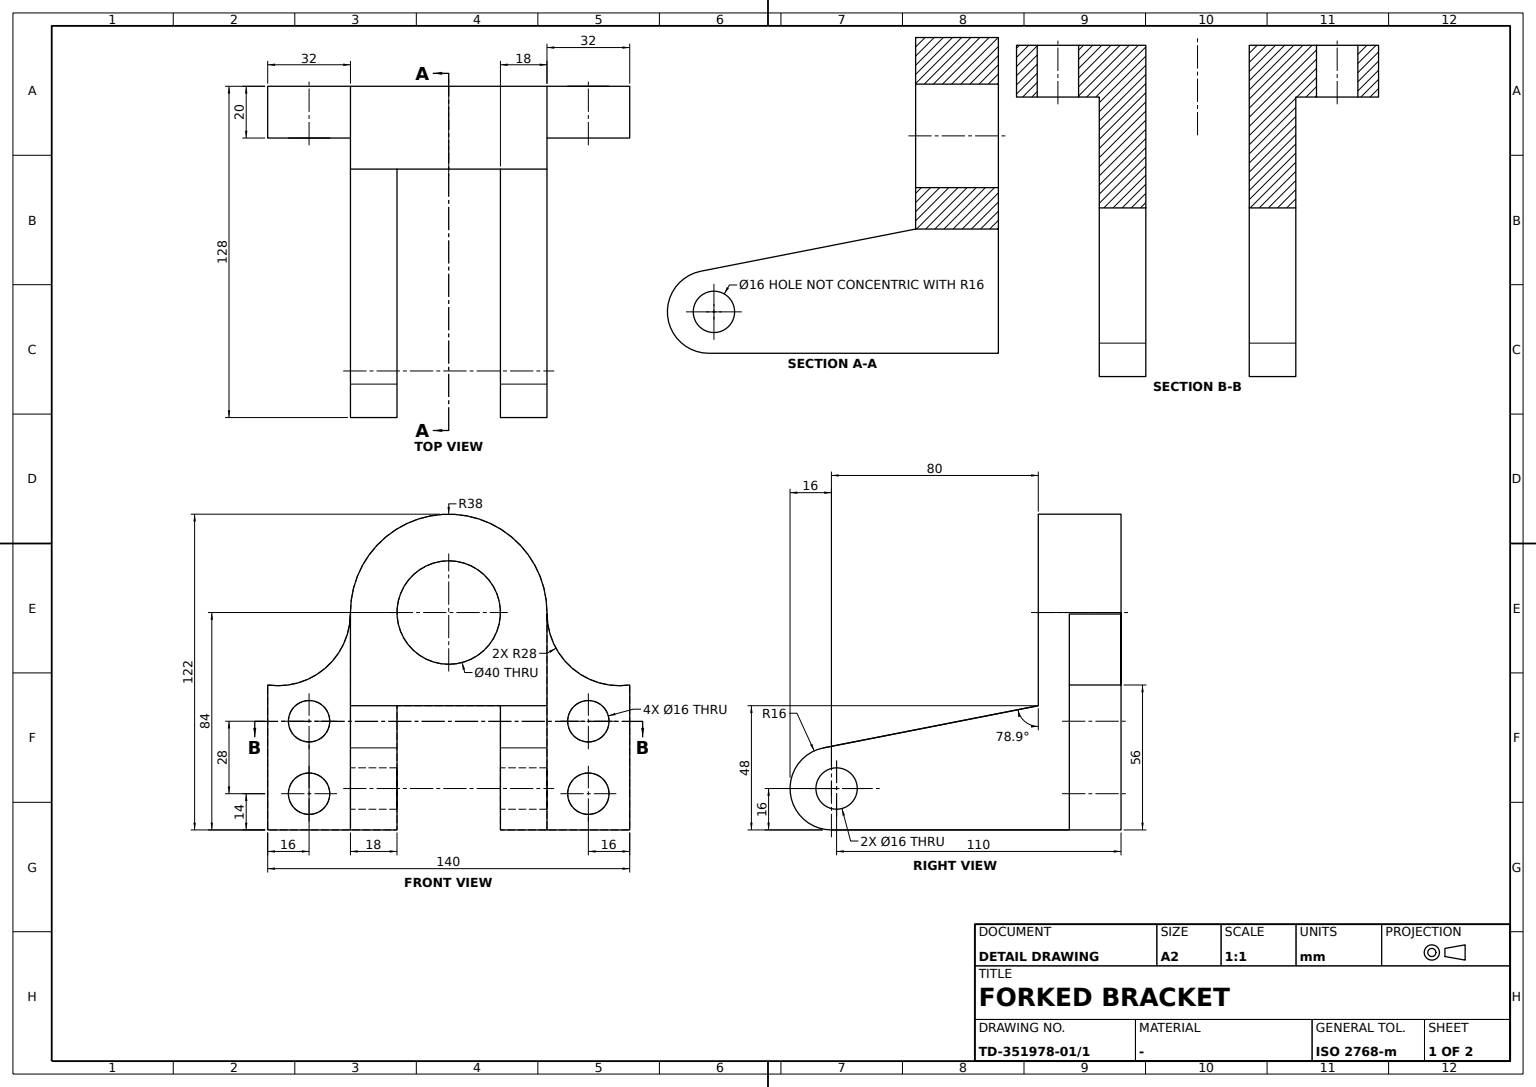
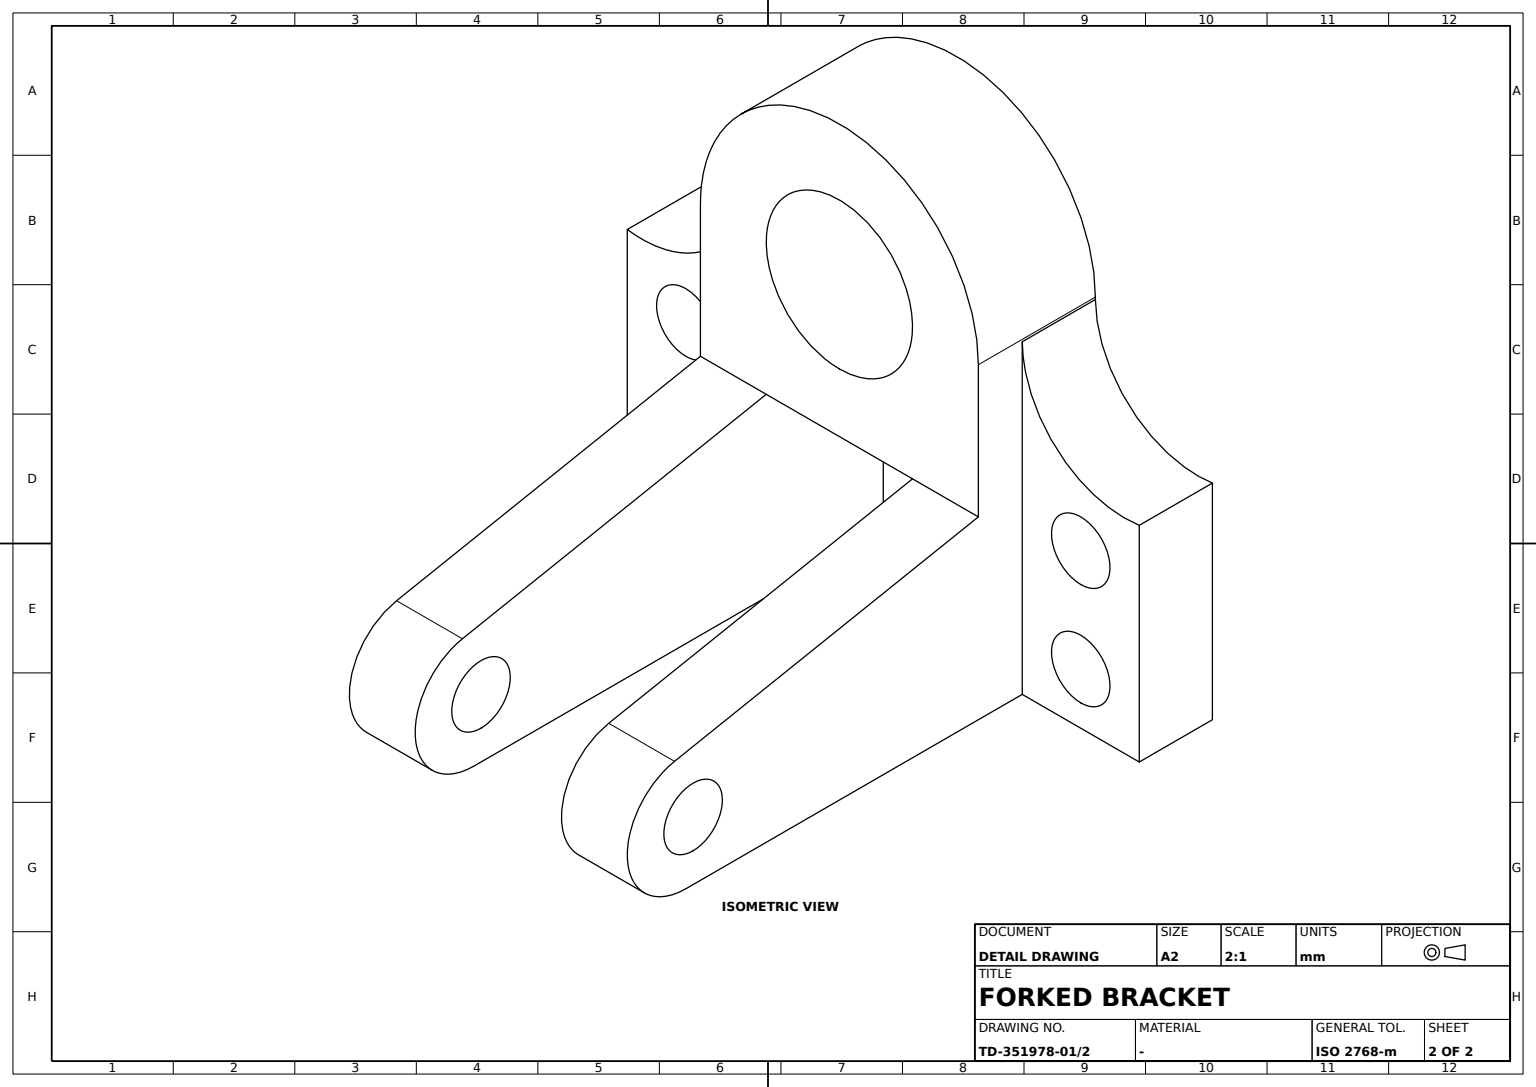
ISO-10303-21;
HEADER;
FILE_DESCRIPTION((''),'2;1');
FILE_NAME('','',(''),(''),'','','');
FILE_SCHEMA(('AUTOMOTIVE_DESIGN'));
ENDSEC;
DATA;
#1=APPLICATION_CONTEXT('');
#2=PRODUCT_CONTEXT('',#1,'mechanical');
#3=PRODUCT('','','',(#2));
#4=PRODUCT_DEFINITION_FORMATION('','',#3);
#5=PRODUCT_DEFINITION_CONTEXT('',#1,'design');
#6=PRODUCT_DEFINITION('','',#4,#5);
#7=PRODUCT_DEFINITION_SHAPE('','',#6);
#8=(LENGTH_UNIT()NAMED_UNIT(*)SI_UNIT(.MILLI.,.METRE.));
#9=(NAMED_UNIT(*)PLANE_ANGLE_UNIT()SI_UNIT($,.RADIAN.));
#10=(NAMED_UNIT(*)SI_UNIT($,.STERADIAN.)SOLID_ANGLE_UNIT());
#11=UNCERTAINTY_MEASURE_WITH_UNIT(LENGTH_MEASURE(0.005),#8,'distance_accuracy_value','');
#12=(GEOMETRIC_REPRESENTATION_CONTEXT(3)GLOBAL_UNCERTAINTY_ASSIGNED_CONTEXT((#11))GLOBAL_UNIT_ASSIGNED_CONTEXT((#8,#9,#10))REPRESENTATION_CONTEXT('',''));
#13=CARTESIAN_POINT('',(94.,-38.,24.));
#14=VERTEX_POINT('',#13);
#15=CARTESIAN_POINT('',(94.,-38.,16.));
#16=DIRECTION('',(0.,1.,0.));
#17=DIRECTION('',(0.,0.,1.));
#18=AXIS2_PLACEMENT_3D('',#15,#16,#17);
#19=CIRCLE('',#18,8.);
#20=EDGE_CURVE('',#14,#14,#19,.F.);
#21=ORIENTED_EDGE('',*,*,#20,.F.);
#22=EDGE_LOOP('',(#21));
#23=FACE_BOUND('',#22,.T.);
#24=CARTESIAN_POINT('',(-16.,-38.,83.425176));
#25=VERTEX_POINT('',#24);
#26=CARTESIAN_POINT('',(-16.,-38.,84.));
#27=VERTEX_POINT('',#26);
#28=CARTESIAN_POINT('',(-16.,-38.,0.));
#29=VECTOR('',#17,1000.);
#30=LINE('',#28,#29);
#31=EDGE_CURVE('',#25,#27,#30,.T.);
#32=ORIENTED_EDGE('',*,*,#31,.F.);
#33=CARTESIAN_POINT('',(4.,-38.,83.425176));
#34=VERTEX_POINT('',#33);
#35=CARTESIAN_POINT('',(-16.,-38.,83.4252));
#36=CARTESIAN_POINT('',(-9.333333,-38.,83.4252));
#37=CARTESIAN_POINT('',(-2.666667,-38.,83.4252));
#38=CARTESIAN_POINT('',(4.,-38.,83.4252));
#39=B_SPLINE_CURVE_WITH_KNOTS('',3,(#35,#36,#37,#38),.UNSPECIFIED.,.F.,.F.,(4,4),(-16.,3.99999975),.UNSPECIFIED.);
#40=EDGE_CURVE('',#25,#34,#39,.T.);
#41=ORIENTED_EDGE('',*,*,#40,.T.);
#42=CARTESIAN_POINT('',(4.,-38.,0.));
#43=VERTEX_POINT('',#42);
#44=DIRECTION('',(0.,0.,-1.));
#45=VECTOR('',#44,1000.);
#46=LINE('',#42,#45);
#47=EDGE_CURVE('',#34,#43,#46,.T.);
#48=ORIENTED_EDGE('',*,*,#47,.T.);
#49=CARTESIAN_POINT('',(96.,-38.,0.));
#50=VERTEX_POINT('',#49);
#51=CARTESIAN_POINT('',(0.,-38.,0.));
#52=DIRECTION('',(1.,0.,0.));
#53=VECTOR('',#52,1000.);
#54=LINE('',#51,#53);
#55=EDGE_CURVE('',#43,#50,#54,.T.);
#56=ORIENTED_EDGE('',*,*,#55,.T.);
#57=CARTESIAN_POINT('',(99.080279,-38.,31.700697));
#58=VERTEX_POINT('',#57);
#59=CARTESIAN_POINT('',(96.,-38.,16.));
#60=AXIS2_PLACEMENT_3D('',#59,#16,#17);
#61=CIRCLE('',#60,16.);
#62=EDGE_CURVE('',#50,#58,#61,.F.);
#63=ORIENTED_EDGE('',*,*,#62,.T.);
#64=CARTESIAN_POINT('',(16.,-38.,48.));
#65=VERTEX_POINT('',#64);
#66=CARTESIAN_POINT('',(9.66098,-38.,49.243636));
#67=DIRECTION('',(-0.981293556,0.,0.192517422));
#68=VECTOR('',#67,1000.);
#69=LINE('',#66,#68);
#70=EDGE_CURVE('',#58,#65,#69,.T.);
#71=ORIENTED_EDGE('',*,*,#70,.T.);
#72=CARTESIAN_POINT('',(16.,-38.,84.));
#73=VERTEX_POINT('',#72);
#74=CARTESIAN_POINT('',(16.,-38.,0.));
#75=LINE('',#74,#29);
#76=EDGE_CURVE('',#65,#73,#75,.T.);
#77=ORIENTED_EDGE('',*,*,#76,.T.);
#78=CARTESIAN_POINT('',(0.,-38.,84.));
#79=LINE('',#78,#53);
#80=EDGE_CURVE('',#73,#27,#79,.F.);
#81=ORIENTED_EDGE('',*,*,#80,.T.);
#82=EDGE_LOOP('',(#32,#41,#48,#56,#63,#71,#77,#81));
#83=FACE_BOUND('',#82,.T.);
#84=AXIS2_PLACEMENT_3D('',#51,#16,#17);
#85=PLANE('',#84);
#86=ADVANCED_FACE('',(#23,#83),#85,.F.);
#87=CARTESIAN_POINT('',(96.,-20.,0.));
#88=VERTEX_POINT('',#87);
#89=CARTESIAN_POINT('',(96.,-29.,0.));
#90=DIRECTION('',(0.,-1.,0.));
#91=VECTOR('',#90,1000.);
#92=LINE('',#89,#91);
#93=EDGE_CURVE('',#50,#88,#92,.F.);
#94=ORIENTED_EDGE('',*,*,#93,.F.);
#95=ORIENTED_EDGE('',*,*,#55,.F.);
#96=CARTESIAN_POINT('',(4.,-70.,0.));
#97=VERTEX_POINT('',#96);
#98=CARTESIAN_POINT('',(4.,-20.,0.));
#99=LINE('',#98,#91);
#100=EDGE_CURVE('',#43,#97,#99,.T.);
#101=ORIENTED_EDGE('',*,*,#100,.T.);
#102=CARTESIAN_POINT('',(-16.,-70.,0.));
#103=VERTEX_POINT('',#102);
#104=LINE('',#102,#53);
#105=EDGE_CURVE('',#103,#97,#104,.T.);
#106=ORIENTED_EDGE('',*,*,#105,.F.);
#107=CARTESIAN_POINT('',(-16.,-20.,0.));
#108=VERTEX_POINT('',#107);
#109=CARTESIAN_POINT('',(-16.,0.,0.));
#110=LINE('',#109,#91);
#111=EDGE_CURVE('',#108,#103,#110,.T.);
#112=ORIENTED_EDGE('',*,*,#111,.F.);
#113=CARTESIAN_POINT('',(0.,-20.,0.));
#114=LINE('',#113,#53);
#115=EDGE_CURVE('',#108,#88,#114,.T.);
#116=ORIENTED_EDGE('',*,*,#115,.T.);
#117=EDGE_LOOP('',(#94,#95,#101,#106,#112,#116));
#118=FACE_BOUND('',#117,.T.);
#119=AXIS2_PLACEMENT_3D('',#113,#17,#90);
#120=PLANE('',#119);
#121=ADVANCED_FACE('',(#118),#120,.F.);
#122=CARTESIAN_POINT('',(99.080279,-20.,31.700697));
#123=VERTEX_POINT('',#122);
#124=CARTESIAN_POINT('',(99.080279,-29.,31.700697));
#125=LINE('',#124,#91);
#126=EDGE_CURVE('',#58,#123,#125,.F.);
#127=ORIENTED_EDGE('',*,*,#126,.T.);
#128=CARTESIAN_POINT('',(16.,-20.,48.));
#129=VERTEX_POINT('',#128);
#130=LINE('',#122,#68);
#131=EDGE_CURVE('',#123,#129,#130,.T.);
#132=ORIENTED_EDGE('',*,*,#131,.T.);
#133=CARTESIAN_POINT('',(16.,0.,48.));
#134=VECTOR('',#16,1000.);
#135=LINE('',#133,#134);
#136=EDGE_CURVE('',#65,#129,#135,.T.);
#137=ORIENTED_EDGE('',*,*,#136,.F.);
#138=ORIENTED_EDGE('',*,*,#70,.F.);
#139=EDGE_LOOP('',(#127,#132,#137,#138));
#140=FACE_BOUND('',#139,.T.);
#141=DIRECTION('',(-0.192517422,0.,-0.981293556));
#142=AXIS2_PLACEMENT_3D('',#57,#141,#67);
#143=PLANE('',#142);
#144=ADVANCED_FACE('',(#140),#143,.F.);
#145=ORIENTED_EDGE('',*,*,#93,.T.);
#146=CARTESIAN_POINT('',(96.,-20.,16.));
#147=AXIS2_PLACEMENT_3D('',#146,#90,#44);
#148=CIRCLE('',#147,16.);
#149=EDGE_CURVE('',#88,#123,#148,.T.);
#150=ORIENTED_EDGE('',*,*,#149,.T.);
#151=ORIENTED_EDGE('',*,*,#126,.F.);
#152=ORIENTED_EDGE('',*,*,#62,.F.);
#153=EDGE_LOOP('',(#145,#150,#151,#152));
#154=FACE_BOUND('',#153,.T.);
#155=CARTESIAN_POINT('',(96.,-29.,16.));
#156=AXIS2_PLACEMENT_3D('',#155,#90,#52);
#157=CYLINDRICAL_SURFACE('',#156,16.);
#158=ADVANCED_FACE('',(#154),#157,.T.);
#159=CARTESIAN_POINT('',(16.,20.,48.));
#160=VERTEX_POINT('',#159);
#161=LINE('',#64,#91);
#162=EDGE_CURVE('',#160,#129,#161,.T.);
#163=ORIENTED_EDGE('',*,*,#162,.T.);
#164=CARTESIAN_POINT('',(-16.,-20.,48.));
#165=VERTEX_POINT('',#164);
#166=CARTESIAN_POINT('',(0.,-20.,48.));
#167=LINE('',#166,#53);
#168=EDGE_CURVE('',#165,#129,#167,.T.);
#169=ORIENTED_EDGE('',*,*,#168,.F.);
#170=CARTESIAN_POINT('',(-16.,20.,48.));
#171=VERTEX_POINT('',#170);
#172=CARTESIAN_POINT('',(-16.,-38.,48.));
#173=LINE('',#172,#91);
#174=EDGE_CURVE('',#171,#165,#173,.T.);
#175=ORIENTED_EDGE('',*,*,#174,.F.);
#176=CARTESIAN_POINT('',(0.,20.,48.));
#177=LINE('',#176,#53);
#178=EDGE_CURVE('',#171,#160,#177,.T.);
#179=ORIENTED_EDGE('',*,*,#178,.T.);
#180=EDGE_LOOP('',(#163,#169,#175,#179));
#181=FACE_BOUND('',#180,.T.);
#182=CARTESIAN_POINT('',(0.,-38.,48.));
#183=AXIS2_PLACEMENT_3D('',#182,#44,#16);
#184=PLANE('',#183);
#185=ADVANCED_FACE('',(#181),#184,.T.);
#186=LINE('',#107,#45);
#187=EDGE_CURVE('',#165,#108,#186,.T.);
#188=ORIENTED_EDGE('',*,*,#187,.F.);
#189=ORIENTED_EDGE('',*,*,#168,.T.);
#190=ORIENTED_EDGE('',*,*,#131,.F.);
#191=ORIENTED_EDGE('',*,*,#149,.F.);
#192=ORIENTED_EDGE('',*,*,#115,.F.);
#193=EDGE_LOOP('',(#188,#189,#190,#191,#192));
#194=FACE_BOUND('',#193,.T.);
#195=CARTESIAN_POINT('',(94.,-20.,8.));
#196=VERTEX_POINT('',#195);
#197=CARTESIAN_POINT('',(94.,-20.,16.));
#198=AXIS2_PLACEMENT_3D('',#197,#90,#44);
#199=CIRCLE('',#198,8.);
#200=EDGE_CURVE('',#196,#196,#199,.T.);
#201=ORIENTED_EDGE('',*,*,#200,.T.);
#202=EDGE_LOOP('',(#201));
#203=FACE_BOUND('',#202,.T.);
#204=AXIS2_PLACEMENT_3D('',#166,#90,#44);
#205=PLANE('',#204);
#206=ADVANCED_FACE('',(#194,#203),#205,.F.);
#207=CARTESIAN_POINT('',(-16.,38.,83.4252));
#208=VERTEX_POINT('',#207);
#209=CARTESIAN_POINT('',(4.,38.,83.425176));
#210=VERTEX_POINT('',#209);
#211=CARTESIAN_POINT('',(4.,38.,83.4252));
#212=CARTESIAN_POINT('',(-2.666667,38.,83.4252));
#213=CARTESIAN_POINT('',(-9.333333,38.,83.4252));
#214=B_SPLINE_CURVE_WITH_KNOTS('',3,(#211,#212,#213,#207),.UNSPECIFIED.,.F.,.F.,(4,4),(-15.99999975,3.999999833),.UNSPECIFIED.);
#215=EDGE_CURVE('',#208,#210,#214,.F.);
#216=ORIENTED_EDGE('',*,*,#215,.T.);
#217=CARTESIAN_POINT('',(4.,70.,55.999787));
#218=VERTEX_POINT('',#217);
#219=CARTESIAN_POINT('',(4.,66.,83.7126));
#220=DIRECTION('',(-1.,0.,0.));
#221=AXIS2_PLACEMENT_3D('',#219,#220,#17);
#222=CIRCLE('',#221,28.);
#223=EDGE_CURVE('',#210,#218,#222,.F.);
#224=ORIENTED_EDGE('',*,*,#223,.T.);
#225=CARTESIAN_POINT('',(-16.,70.,55.999787));
#226=VERTEX_POINT('',#225);
#227=LINE('',#225,#53);
#228=EDGE_CURVE('',#226,#218,#227,.T.);
#229=ORIENTED_EDGE('',*,*,#228,.F.);
#230=CARTESIAN_POINT('',(-16.,66.,83.7126));
#231=AXIS2_PLACEMENT_3D('',#230,#52,#44);
#232=CIRCLE('',#231,28.);
#233=EDGE_CURVE('',#208,#226,#232,.T.);
#234=ORIENTED_EDGE('',*,*,#233,.F.);
#235=EDGE_LOOP('',(#216,#224,#229,#234));
#236=FACE_BOUND('',#235,.T.);
#237=CARTESIAN_POINT('',(-6.,66.,83.7126));
#238=AXIS2_PLACEMENT_3D('',#237,#52,#16);
#239=CYLINDRICAL_SURFACE('',#238,28.);
#240=ADVANCED_FACE('',(#236),#239,.F.);
#241=CARTESIAN_POINT('',(4.,54.,22.));
#242=VERTEX_POINT('',#241);
#243=CARTESIAN_POINT('',(4.,54.,14.));
#244=AXIS2_PLACEMENT_3D('',#243,#220,#17);
#245=CIRCLE('',#244,8.);
#246=EDGE_CURVE('',#242,#242,#245,.T.);
#247=ORIENTED_EDGE('',*,*,#246,.F.);
#248=EDGE_LOOP('',(#247));
#249=FACE_BOUND('',#248,.T.);
#250=CARTESIAN_POINT('',(-16.,54.,6.));
#251=VERTEX_POINT('',#250);
#252=CARTESIAN_POINT('',(-16.,54.,14.));
#253=AXIS2_PLACEMENT_3D('',#252,#52,#44);
#254=CIRCLE('',#253,8.);
#255=EDGE_CURVE('',#251,#251,#254,.F.);
#256=ORIENTED_EDGE('',*,*,#255,.T.);
#257=EDGE_LOOP('',(#256));
#258=FACE_BOUND('',#257,.T.);
#259=CARTESIAN_POINT('',(-6.,54.,14.));
#260=AXIS2_PLACEMENT_3D('',#259,#220,#90);
#261=CYLINDRICAL_SURFACE('',#260,8.);
#262=ADVANCED_FACE('',(#249,#258),#261,.F.);
#263=CARTESIAN_POINT('',(96.,20.,0.));
#264=VERTEX_POINT('',#263);
#265=CARTESIAN_POINT('',(99.080279,20.,31.700697));
#266=VERTEX_POINT('',#265);
#267=CARTESIAN_POINT('',(96.,20.,16.));
#268=AXIS2_PLACEMENT_3D('',#267,#16,#17);
#269=CIRCLE('',#268,16.);
#270=EDGE_CURVE('',#264,#266,#269,.F.);
#271=ORIENTED_EDGE('',*,*,#270,.F.);
#272=CARTESIAN_POINT('',(96.,38.,0.));
#273=VERTEX_POINT('',#272);
#274=EDGE_CURVE('',#273,#264,#92,.T.);
#275=ORIENTED_EDGE('',*,*,#274,.F.);
#276=CARTESIAN_POINT('',(99.080279,38.,31.700697));
#277=VERTEX_POINT('',#276);
#278=CARTESIAN_POINT('',(96.,38.,16.));
#279=AXIS2_PLACEMENT_3D('',#278,#90,#44);
#280=CIRCLE('',#279,16.);
#281=EDGE_CURVE('',#273,#277,#280,.T.);
#282=ORIENTED_EDGE('',*,*,#281,.T.);
#283=EDGE_CURVE('',#277,#266,#125,.T.);
#284=ORIENTED_EDGE('',*,*,#283,.T.);
#285=EDGE_LOOP('',(#271,#275,#282,#284));
#286=FACE_BOUND('',#285,.T.);
#287=ADVANCED_FACE('',(#286),#157,.T.);
#288=ORIENTED_EDGE('',*,*,#105,.T.);
#289=CARTESIAN_POINT('',(4.,-70.,55.999787));
#290=VERTEX_POINT('',#289);
#291=LINE('',#96,#29);
#292=EDGE_CURVE('',#97,#290,#291,.T.);
#293=ORIENTED_EDGE('',*,*,#292,.T.);
#294=CARTESIAN_POINT('',(-16.,-70.,55.999787));
#295=VERTEX_POINT('',#294);
#296=VECTOR('',#220,1000.);
#297=LINE('',#294,#296);
#298=EDGE_CURVE('',#295,#290,#297,.F.);
#299=ORIENTED_EDGE('',*,*,#298,.F.);
#300=LINE('',#102,#29);
#301=EDGE_CURVE('',#103,#295,#300,.T.);
#302=ORIENTED_EDGE('',*,*,#301,.F.);
#303=EDGE_LOOP('',(#288,#293,#299,#302));
#304=FACE_BOUND('',#303,.T.);
#305=AXIS2_PLACEMENT_3D('',#102,#16,#17);
#306=PLANE('',#305);
#307=ADVANCED_FACE('',(#304),#306,.F.);
#308=CARTESIAN_POINT('',(94.,20.,24.));
#309=VERTEX_POINT('',#308);
#310=CARTESIAN_POINT('',(94.,20.,16.));
#311=AXIS2_PLACEMENT_3D('',#310,#16,#17);
#312=CIRCLE('',#311,8.);
#313=EDGE_CURVE('',#309,#309,#312,.T.);
#314=ORIENTED_EDGE('',*,*,#313,.F.);
#315=EDGE_LOOP('',(#314));
#316=FACE_BOUND('',#315,.T.);
#317=CARTESIAN_POINT('',(94.,38.,8.));
#318=VERTEX_POINT('',#317);
#319=CARTESIAN_POINT('',(94.,38.,16.));
#320=AXIS2_PLACEMENT_3D('',#319,#90,#44);
#321=CIRCLE('',#320,8.);
#322=EDGE_CURVE('',#318,#318,#321,.T.);
#323=ORIENTED_EDGE('',*,*,#322,.F.);
#324=EDGE_LOOP('',(#323));
#325=FACE_BOUND('',#324,.T.);
#326=CARTESIAN_POINT('',(94.,6.5,16.));
#327=AXIS2_PLACEMENT_3D('',#326,#90,#52);
#328=CYLINDRICAL_SURFACE('',#327,8.);
#329=ADVANCED_FACE('',(#316,#325),#328,.F.);
#330=CARTESIAN_POINT('',(-16.,54.,34.));
#331=VERTEX_POINT('',#330);
#332=CARTESIAN_POINT('',(-16.,54.,42.));
#333=AXIS2_PLACEMENT_3D('',#332,#52,#44);
#334=CIRCLE('',#333,8.);
#335=EDGE_CURVE('',#331,#331,#334,.F.);
#336=ORIENTED_EDGE('',*,*,#335,.T.);
#337=EDGE_LOOP('',(#336));
#338=FACE_BOUND('',#337,.T.);
#339=CARTESIAN_POINT('',(4.,54.,50.));
#340=VERTEX_POINT('',#339);
#341=CARTESIAN_POINT('',(4.,54.,42.));
#342=AXIS2_PLACEMENT_3D('',#341,#220,#17);
#343=CIRCLE('',#342,8.);
#344=EDGE_CURVE('',#340,#340,#343,.T.);
#345=ORIENTED_EDGE('',*,*,#344,.F.);
#346=EDGE_LOOP('',(#345));
#347=FACE_BOUND('',#346,.T.);
#348=CARTESIAN_POINT('',(-6.,54.,42.));
#349=AXIS2_PLACEMENT_3D('',#348,#220,#90);
#350=CYLINDRICAL_SURFACE('',#349,8.);
#351=ADVANCED_FACE('',(#338,#347),#350,.F.);
#352=CARTESIAN_POINT('',(16.,0.,64.));
#353=VERTEX_POINT('',#352);
#354=CARTESIAN_POINT('',(16.,0.,84.));
#355=AXIS2_PLACEMENT_3D('',#354,#52,#44);
#356=CIRCLE('',#355,20.);
#357=EDGE_CURVE('',#353,#353,#356,.T.);
#358=ORIENTED_EDGE('',*,*,#357,.T.);
#359=EDGE_LOOP('',(#358));
#360=FACE_BOUND('',#359,.T.);
#361=CARTESIAN_POINT('',(-16.,0.,64.));
#362=VERTEX_POINT('',#361);
#363=CARTESIAN_POINT('',(-16.,0.,84.));
#364=AXIS2_PLACEMENT_3D('',#363,#52,#44);
#365=CIRCLE('',#364,20.);
#366=EDGE_CURVE('',#362,#362,#365,.T.);
#367=ORIENTED_EDGE('',*,*,#366,.F.);
#368=EDGE_LOOP('',(#367));
#369=FACE_BOUND('',#368,.T.);
#370=CARTESIAN_POINT('',(0.,0.,84.));
#371=AXIS2_PLACEMENT_3D('',#370,#52,#16);
#372=CYLINDRICAL_SURFACE('',#371,20.);
#373=ADVANCED_FACE('',(#360,#369),#372,.F.);
#374=CARTESIAN_POINT('',(16.,38.,48.));
#375=VERTEX_POINT('',#374);
#376=EDGE_CURVE('',#375,#160,#161,.T.);
#377=ORIENTED_EDGE('',*,*,#376,.T.);
#378=CARTESIAN_POINT('',(9.66098,20.,49.243636));
#379=LINE('',#378,#68);
#380=EDGE_CURVE('',#266,#160,#379,.T.);
#381=ORIENTED_EDGE('',*,*,#380,.F.);
#382=ORIENTED_EDGE('',*,*,#283,.F.);
#383=LINE('',#276,#68);
#384=EDGE_CURVE('',#277,#375,#383,.T.);
#385=ORIENTED_EDGE('',*,*,#384,.T.);
#386=EDGE_LOOP('',(#377,#381,#382,#385));
#387=FACE_BOUND('',#386,.T.);
#388=ADVANCED_FACE('',(#387),#143,.F.);
#389=CARTESIAN_POINT('',(-16.,70.,0.));
#390=VERTEX_POINT('',#389);
#391=CARTESIAN_POINT('',(4.,70.,0.));
#392=VERTEX_POINT('',#391);
#393=LINE('',#389,#53);
#394=EDGE_CURVE('',#390,#392,#393,.T.);
#395=ORIENTED_EDGE('',*,*,#394,.F.);
#396=LINE('',#389,#29);
#397=EDGE_CURVE('',#390,#226,#396,.T.);
#398=ORIENTED_EDGE('',*,*,#397,.T.);
#399=ORIENTED_EDGE('',*,*,#228,.T.);
#400=LINE('',#391,#29);
#401=EDGE_CURVE('',#392,#218,#400,.T.);
#402=ORIENTED_EDGE('',*,*,#401,.F.);
#403=EDGE_LOOP('',(#395,#398,#399,#402));
#404=FACE_BOUND('',#403,.T.);
#405=AXIS2_PLACEMENT_3D('',#389,#16,#17);
#406=PLANE('',#405);
#407=ADVANCED_FACE('',(#404),#406,.T.);
#408=CARTESIAN_POINT('',(4.,38.,0.));
#409=VERTEX_POINT('',#408);
#410=CARTESIAN_POINT('',(4.,38.,48.));
#411=LINE('',#410,#45);
#412=EDGE_CURVE('',#210,#409,#411,.T.);
#413=ORIENTED_EDGE('',*,*,#412,.T.);
#414=CARTESIAN_POINT('',(4.,0.,0.));
#415=LINE('',#414,#134);
#416=EDGE_CURVE('',#409,#392,#415,.T.);
#417=ORIENTED_EDGE('',*,*,#416,.T.);
#418=ORIENTED_EDGE('',*,*,#401,.T.);
#419=ORIENTED_EDGE('',*,*,#223,.F.);
#420=EDGE_LOOP('',(#413,#417,#418,#419));
#421=FACE_BOUND('',#420,.T.);
#422=ORIENTED_EDGE('',*,*,#344,.T.);
#423=EDGE_LOOP('',(#422));
#424=FACE_BOUND('',#423,.T.);
#425=ORIENTED_EDGE('',*,*,#246,.T.);
#426=EDGE_LOOP('',(#425));
#427=FACE_BOUND('',#426,.T.);
#428=AXIS2_PLACEMENT_3D('',#414,#220,#90);
#429=PLANE('',#428);
#430=ADVANCED_FACE('',(#421,#424,#427),#429,.F.);
#431=ORIENTED_EDGE('',*,*,#274,.T.);
#432=CARTESIAN_POINT('',(-16.,20.,0.));
#433=VERTEX_POINT('',#432);
#434=CARTESIAN_POINT('',(0.,20.,0.));
#435=LINE('',#434,#53);
#436=EDGE_CURVE('',#433,#264,#435,.T.);
#437=ORIENTED_EDGE('',*,*,#436,.F.);
#438=EDGE_CURVE('',#390,#433,#110,.T.);
#439=ORIENTED_EDGE('',*,*,#438,.F.);
#440=ORIENTED_EDGE('',*,*,#394,.T.);
#441=ORIENTED_EDGE('',*,*,#416,.F.);
#442=CARTESIAN_POINT('',(0.,38.,0.));
#443=LINE('',#442,#53);
#444=EDGE_CURVE('',#409,#273,#443,.T.);
#445=ORIENTED_EDGE('',*,*,#444,.T.);
#446=EDGE_LOOP('',(#431,#437,#439,#440,#441,#445));
#447=FACE_BOUND('',#446,.T.);
#448=ADVANCED_FACE('',(#447),#120,.F.);
#449=ORIENTED_EDGE('',*,*,#40,.F.);
#450=CARTESIAN_POINT('',(-16.,-66.,83.7126));
#451=AXIS2_PLACEMENT_3D('',#450,#52,#44);
#452=CIRCLE('',#451,28.);
#453=EDGE_CURVE('',#25,#295,#452,.F.);
#454=ORIENTED_EDGE('',*,*,#453,.T.);
#455=ORIENTED_EDGE('',*,*,#298,.T.);
#456=CARTESIAN_POINT('',(4.,-66.,83.7126));
#457=AXIS2_PLACEMENT_3D('',#456,#220,#17);
#458=CIRCLE('',#457,28.);
#459=EDGE_CURVE('',#34,#290,#458,.T.);
#460=ORIENTED_EDGE('',*,*,#459,.F.);
#461=EDGE_LOOP('',(#449,#454,#455,#460));
#462=FACE_BOUND('',#461,.T.);
#463=CARTESIAN_POINT('',(-6.,-66.,83.7126));
#464=AXIS2_PLACEMENT_3D('',#463,#220,#90);
#465=CYLINDRICAL_SURFACE('',#464,28.);
#466=ADVANCED_FACE('',(#462),#465,.F.);
#467=ORIENTED_EDGE('',*,*,#162,.F.);
#468=ORIENTED_EDGE('',*,*,#376,.F.);
#469=CARTESIAN_POINT('',(16.,38.,84.));
#470=VERTEX_POINT('',#469);
#471=CARTESIAN_POINT('',(16.,38.,0.));
#472=LINE('',#471,#45);
#473=EDGE_CURVE('',#470,#375,#472,.T.);
#474=ORIENTED_EDGE('',*,*,#473,.F.);
#475=CIRCLE('',#355,38.);
#476=EDGE_CURVE('',#470,#73,#475,.T.);
#477=ORIENTED_EDGE('',*,*,#476,.T.);
#478=ORIENTED_EDGE('',*,*,#76,.F.);
#479=ORIENTED_EDGE('',*,*,#136,.T.);
#480=EDGE_LOOP('',(#467,#468,#474,#477,#478,#479));
#481=FACE_BOUND('',#480,.T.);
#482=ORIENTED_EDGE('',*,*,#357,.F.);
#483=EDGE_LOOP('',(#482));
#484=FACE_BOUND('',#483,.T.);
#485=CARTESIAN_POINT('',(16.,0.,0.));
#486=AXIS2_PLACEMENT_3D('',#485,#52,#16);
#487=PLANE('',#486);
#488=ADVANCED_FACE('',(#481,#484),#487,.T.);
#489=ORIENTED_EDGE('',*,*,#80,.F.);
#490=ORIENTED_EDGE('',*,*,#476,.F.);
#491=CARTESIAN_POINT('',(-16.,38.,84.));
#492=VERTEX_POINT('',#491);
#493=CARTESIAN_POINT('',(0.,38.,84.));
#494=LINE('',#493,#53);
#495=EDGE_CURVE('',#470,#492,#494,.F.);
#496=ORIENTED_EDGE('',*,*,#495,.T.);
#497=CIRCLE('',#364,38.);
#498=EDGE_CURVE('',#492,#27,#497,.T.);
#499=ORIENTED_EDGE('',*,*,#498,.T.);
#500=EDGE_LOOP('',(#489,#490,#496,#499));
#501=FACE_BOUND('',#500,.T.);
#502=CYLINDRICAL_SURFACE('',#371,38.);
#503=ADVANCED_FACE('',(#501),#502,.T.);
#504=ORIENTED_EDGE('',*,*,#495,.F.);
#505=ORIENTED_EDGE('',*,*,#473,.T.);
#506=ORIENTED_EDGE('',*,*,#384,.F.);
#507=ORIENTED_EDGE('',*,*,#281,.F.);
#508=ORIENTED_EDGE('',*,*,#444,.F.);
#509=ORIENTED_EDGE('',*,*,#412,.F.);
#510=ORIENTED_EDGE('',*,*,#215,.F.);
#511=CARTESIAN_POINT('',(-16.,38.,0.));
#512=LINE('',#511,#45);
#513=EDGE_CURVE('',#492,#208,#512,.T.);
#514=ORIENTED_EDGE('',*,*,#513,.F.);
#515=EDGE_LOOP('',(#504,#505,#506,#507,#508,#509,#510,#514));
#516=FACE_BOUND('',#515,.T.);
#517=ORIENTED_EDGE('',*,*,#322,.T.);
#518=EDGE_LOOP('',(#517));
#519=FACE_BOUND('',#518,.T.);
#520=CARTESIAN_POINT('',(0.,38.,48.));
#521=AXIS2_PLACEMENT_3D('',#520,#90,#44);
#522=PLANE('',#521);
#523=ADVANCED_FACE('',(#516,#519),#522,.F.);
#524=ORIENTED_EDGE('',*,*,#255,.F.);
#525=EDGE_LOOP('',(#524));
#526=FACE_BOUND('',#525,.T.);
#527=ORIENTED_EDGE('',*,*,#513,.T.);
#528=ORIENTED_EDGE('',*,*,#233,.T.);
#529=ORIENTED_EDGE('',*,*,#397,.F.);
#530=ORIENTED_EDGE('',*,*,#438,.T.);
#531=LINE('',#432,#29);
#532=EDGE_CURVE('',#433,#171,#531,.T.);
#533=ORIENTED_EDGE('',*,*,#532,.T.);
#534=ORIENTED_EDGE('',*,*,#174,.T.);
#535=ORIENTED_EDGE('',*,*,#187,.T.);
#536=ORIENTED_EDGE('',*,*,#111,.T.);
#537=ORIENTED_EDGE('',*,*,#301,.T.);
#538=ORIENTED_EDGE('',*,*,#453,.F.);
#539=ORIENTED_EDGE('',*,*,#31,.T.);
#540=ORIENTED_EDGE('',*,*,#498,.F.);
#541=EDGE_LOOP('',(#527,#528,#529,#530,#533,#534,#535,#536,#537,#538,#539,#540));
#542=FACE_BOUND('',#541,.T.);
#543=CARTESIAN_POINT('',(-16.,-54.,6.));
#544=VERTEX_POINT('',#543);
#545=CARTESIAN_POINT('',(-16.,-54.,14.));
#546=AXIS2_PLACEMENT_3D('',#545,#52,#44);
#547=CIRCLE('',#546,8.);
#548=EDGE_CURVE('',#544,#544,#547,.T.);
#549=ORIENTED_EDGE('',*,*,#548,.T.);
#550=EDGE_LOOP('',(#549));
#551=FACE_BOUND('',#550,.T.);
#552=ORIENTED_EDGE('',*,*,#335,.F.);
#553=EDGE_LOOP('',(#552));
#554=FACE_BOUND('',#553,.T.);
#555=CARTESIAN_POINT('',(-16.,-54.,34.));
#556=VERTEX_POINT('',#555);
#557=CARTESIAN_POINT('',(-16.,-54.,42.));
#558=AXIS2_PLACEMENT_3D('',#557,#52,#44);
#559=CIRCLE('',#558,8.);
#560=EDGE_CURVE('',#556,#556,#559,.T.);
#561=ORIENTED_EDGE('',*,*,#560,.T.);
#562=EDGE_LOOP('',(#561));
#563=FACE_BOUND('',#562,.T.);
#564=ORIENTED_EDGE('',*,*,#366,.T.);
#565=EDGE_LOOP('',(#564));
#566=FACE_BOUND('',#565,.T.);
#567=AXIS2_PLACEMENT_3D('',#109,#52,#16);
#568=PLANE('',#567);
#569=ADVANCED_FACE('',(#526,#542,#551,#554,#563,#566),#568,.F.);
#570=ORIENTED_EDGE('',*,*,#200,.F.);
#571=EDGE_LOOP('',(#570));
#572=FACE_BOUND('',#571,.T.);
#573=ORIENTED_EDGE('',*,*,#20,.T.);
#574=EDGE_LOOP('',(#573));
#575=FACE_BOUND('',#574,.T.);
#576=ADVANCED_FACE('',(#572,#575),#328,.F.);
#577=ORIENTED_EDGE('',*,*,#560,.F.);
#578=EDGE_LOOP('',(#577));
#579=FACE_BOUND('',#578,.T.);
#580=CARTESIAN_POINT('',(4.,-54.,50.));
#581=VERTEX_POINT('',#580);
#582=CARTESIAN_POINT('',(4.,-54.,42.));
#583=AXIS2_PLACEMENT_3D('',#582,#220,#17);
#584=CIRCLE('',#583,8.);
#585=EDGE_CURVE('',#581,#581,#584,.F.);
#586=ORIENTED_EDGE('',*,*,#585,.T.);
#587=EDGE_LOOP('',(#586));
#588=FACE_BOUND('',#587,.T.);
#589=CARTESIAN_POINT('',(-6.,-54.,42.));
#590=AXIS2_PLACEMENT_3D('',#589,#52,#16);
#591=CYLINDRICAL_SURFACE('',#590,8.);
#592=ADVANCED_FACE('',(#579,#588),#591,.F.);
#593=ORIENTED_EDGE('',*,*,#548,.F.);
#594=EDGE_LOOP('',(#593));
#595=FACE_BOUND('',#594,.T.);
#596=CARTESIAN_POINT('',(4.,-54.,22.));
#597=VERTEX_POINT('',#596);
#598=CARTESIAN_POINT('',(4.,-54.,14.));
#599=AXIS2_PLACEMENT_3D('',#598,#220,#17);
#600=CIRCLE('',#599,8.);
#601=EDGE_CURVE('',#597,#597,#600,.F.);
#602=ORIENTED_EDGE('',*,*,#601,.T.);
#603=EDGE_LOOP('',(#602));
#604=FACE_BOUND('',#603,.T.);
#605=CARTESIAN_POINT('',(-6.,-54.,14.));
#606=AXIS2_PLACEMENT_3D('',#605,#52,#16);
#607=CYLINDRICAL_SURFACE('',#606,8.);
#608=ADVANCED_FACE('',(#595,#604),#607,.F.);
#609=ORIENTED_EDGE('',*,*,#585,.F.);
#610=EDGE_LOOP('',(#609));
#611=FACE_BOUND('',#610,.T.);
#612=ORIENTED_EDGE('',*,*,#601,.F.);
#613=EDGE_LOOP('',(#612));
#614=FACE_BOUND('',#613,.T.);
#615=ORIENTED_EDGE('',*,*,#100,.F.);
#616=ORIENTED_EDGE('',*,*,#47,.F.);
#617=ORIENTED_EDGE('',*,*,#459,.T.);
#618=ORIENTED_EDGE('',*,*,#292,.F.);
#619=EDGE_LOOP('',(#615,#616,#617,#618));
#620=FACE_BOUND('',#619,.T.);
#621=ADVANCED_FACE('',(#611,#614,#620),#429,.F.);
#622=ORIENTED_EDGE('',*,*,#313,.T.);
#623=EDGE_LOOP('',(#622));
#624=FACE_BOUND('',#623,.T.);
#625=ORIENTED_EDGE('',*,*,#380,.T.);
#626=ORIENTED_EDGE('',*,*,#178,.F.);
#627=ORIENTED_EDGE('',*,*,#532,.F.);
#628=ORIENTED_EDGE('',*,*,#436,.T.);
#629=ORIENTED_EDGE('',*,*,#270,.T.);
#630=EDGE_LOOP('',(#625,#626,#627,#628,#629));
#631=FACE_BOUND('',#630,.T.);
#632=AXIS2_PLACEMENT_3D('',#434,#16,#17);
#633=PLANE('',#632);
#634=ADVANCED_FACE('',(#624,#631),#633,.F.);
#635=CLOSED_SHELL('',(#86,#121,#144,#158,#185,#206,#240,#262,#287,#307,#329,#351,#373,#388,#407,#430,#448,#466,#488,#503,#523,#569,#576,#592,#608,#621,#634));
#636=MANIFOLD_SOLID_BREP('',#635);
#637=ADVANCED_BREP_SHAPE_REPRESENTATION('',(#636),#12);
#638=SHAPE_DEFINITION_REPRESENTATION(#7,#637);
ENDSEC;
END-ISO-10303-21;
